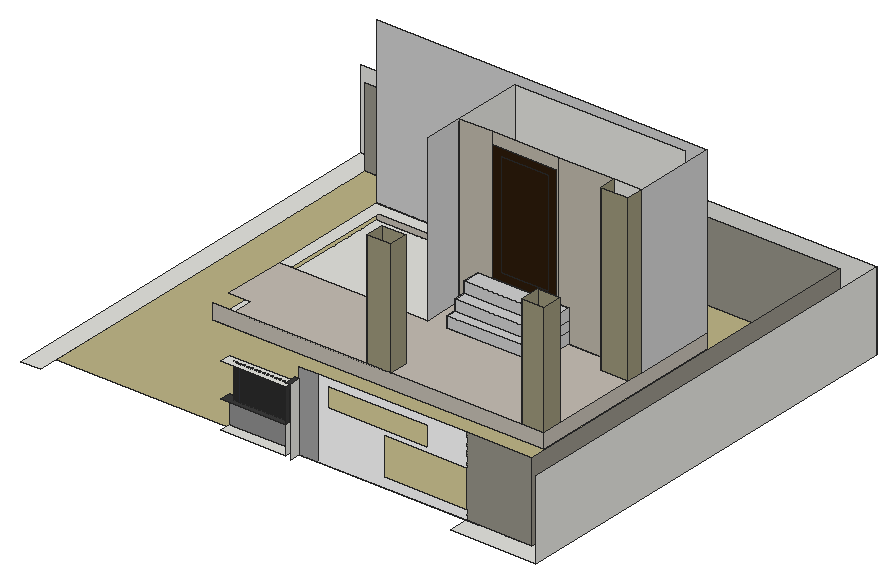
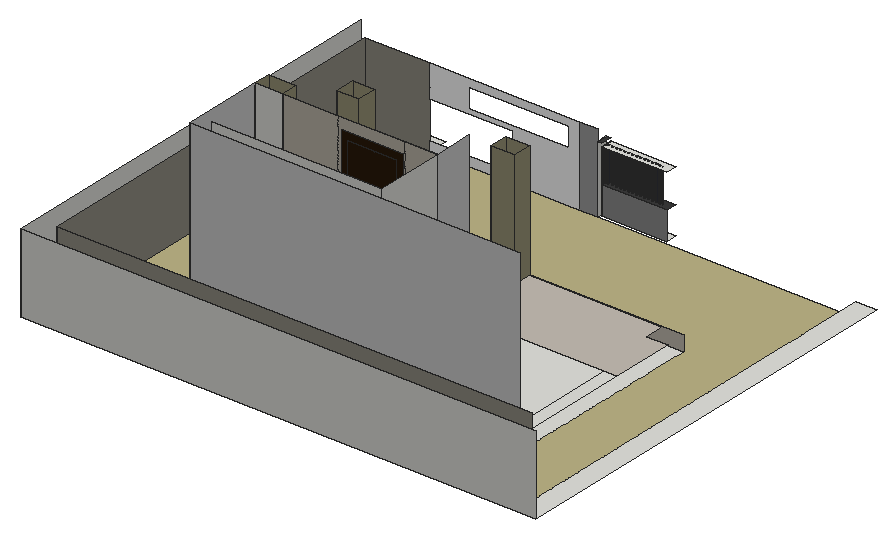
# SketchUp Ruby script. Lengths in inches.
U = 1.inch
M = Sketchup.active_model
def pt(a) = Geom::Point3d.new(a.map { |v| v * U })
def face(e, loops, mat)
  f = e.add_face(loops[0].map { |a| pt(a) })
  loops[1..].each { |l| e.add_face(l.map { |a| pt(a) }).erase! }
  f.material = f.back_material = mat if mat
  f
end
# faces: each face lists its corners as indices into pts; further lists are holes
def faces(e, pts, list, mat = nil) = list.each { |f| face(e, (f[0].is_a?(Array) ? f : [f]).map { |l| l.map { |i| pts[i] } }, mat) }
# xy, xz, yz: faces in a plane at the given z, y or x. An outline is a flat list of corners, or four numbers for a rectangle; further outlines are holes
def ring(l) = l.size == 4 ? [[l[0], l[1]], [l[2], l[1]], [l[2], l[3]], [l[0], l[3]]] : l.each_slice(2).to_a
def flat(e, list, mat, &to3) = list.each { |f| face(e, (f[0].is_a?(Array) ? f : [f]).map { |l| ring(l).map { |u, v| to3.(u, v) } }, mat) }
def xy(e, z, list, mat = nil) = flat(e, list, mat) { |x, y| [x, y, z] }
def xz(e, y, list, mat = nil) = flat(e, list, mat) { |x, z| [x, y, z] }
def yz(e, x, list, mat = nil) = flat(e, list, mat) { |y, z| [x, y, z] }
def lines(e, pts, list) = list.each { |a, b| e.add_line(pt(pts[a]), pt(pts[b])) }
# prism: a flat outline (further loops are holes) pulled along v
def prism(e, loops, v, mat = nil)
  f = face(e, loops, mat); d = Geom::Vector3d.new(v.map { |x| x * U })
  f.pushpull(f.normal.samedirection?(d) ? d.length : -d.length)
end
def box(e, o, s, mat = nil) = prism(e, [[o, [o[0] + s[0], o[1], o[2]], [o[0] + s[0], o[1] + s[1], o[2]], [o[0], o[1] + s[1], o[2]]]], [0, 0, s[2]], mat)
def at(x, y, z, deg = 0) = Geom::Transformation.translation(pt([x, y, z])) * Geom::Transformation.rotation(ORIGIN, Z_AXIS, deg.degrees)
def axes(o, x, y, z) = Geom::Transformation.new([*x, 0, *y, 0, *z, 0, *pt(o).to_a, 1])
def part(name) = M.definitions.add(name)
# library, detail: a bought-in or finely detailed component or shape, given as its bounding box
def library(name, o, s) = part(name).tap { |d| box(d.entities, o, s) }
def detail(e, o, s) = box(e.add_group.entities, o, s)
def put(e, d, t, mat = nil) = e.add_instance(d, t).tap { |i| i.material = mat if mat }
def group(e, t, mat = nil) = e.add_group.tap { |g| g.transformation = t; g.material = mat if mat }.entities
root = M.entities
M.materials.add("[Blinds Vertical Stripe Gray]").color = [160, 160, 160]
M.materials.add("[Blinds Vertical Stripe Gray]1").color = [252, 252, 252]
M.materials.add("[Carrera Marble]").color = [207, 207, 207]
M.materials.add("[Cinder Block]").color = [191, 184, 171]
M.materials.add("[Cladding Siding White]").color = [207, 207, 207]
M.materials.add("[Color M04]").color = [142, 142, 142]
M.materials.add("[Color M07]").color = [58, 58, 58]
M.materials.add("[Field Rectangle Tile]").color = [196, 189, 179]
M.materials.add("[Formica Graystone]").color = [149, 146, 135]
M.materials.add("[Formica Laminate Dark]").color = [50, 53, 60]
M.materials.add("[Stone Coursed Rough]").color = [155, 150, 122]
M.materials.add("[Tile Ceramic Natural]").color = [189, 180, 134]
M.materials.add("[Wood Floor Parquet]").color = [45, 28, 12]
xy(root,0,[[0,96.24,0,408.18,377.8125,408.18,377.8125,96.24,315.3,96.24,315.3,111,363.05,111,363.05,393.42,14.76,393.42,14.76,96.24],[55.77,203.17,297.85,352.92]])
xy(root,0,[[[14.76,111,363.05,393.42],[55.77,203.17,297.85,352.92]]],"[Tile Ceramic Natural]")
xy(root,1.75,[[141.86,102.91,189.5,111]])
xy(root,10.875,[[168.55,203.17,186.24,216.5],[281.86,203.17,297.85,217.98],[55.77,263.99,55.77,352.92,297.85,352.92,297.85,292.92,288.72,292.92,288.72,343.79,64.9,343.79,64.9,263.99],[178.12,264.54,244.68,292.92],[277.86,280.61,288.72,292.92],
  [288.72,280.61,297.85,292.92],[164.37,292.92,288.72,343.79]])
xy(root,10.875,[[71.76,203.17,168.55,203.17,168.55,216.5,186.24,216.5,186.24,203.17,281.86,203.17,281.86,217.98,297.85,217.98,297.85,280.61,277.86,280.61,277.86,292.92,244.68,292.92,244.68,264.54,178.12,264.54,178.12,292.92,164.37,292.92,164.37,263.99,55.77,263.99,55.77,217.98,71.76,217.98]],"[Field Rectangle Tile]")
xy(root,18.65,[[178.12,271.92,244.68,292.92]])
xy(root,18.65,[[178.12,264.54,244.68,271.92]],"[Carrera Marble]")
xy(root,22.1875,[[[141.86,102.91,189.5,111],[144.08,106,143.9,106.02,143.74,106.09,143.6,106.2,143.49,106.34,143.42,106.51,143.4,106.6875,143.42,106.87,143.49,107.03,143.6,107.17,143.74,107.28,143.9,107.35,144.08,107.375,144.26,107.35,144.43,107.28,144.57,107.17,144.68,107.03,144.75,106.87,144.77,106.6875,144.75,106.51,144.68,106.34,144.57,106.2,144.43,106.09,144.26,106.02],[146.96,106,146.78,106.02,146.61,106.09,146.47,106.2,146.36,106.34,146.29,106.51,146.27,106.6875,146.29,106.87,146.36,107.03,146.47,107.17,146.61,107.28,146.78,107.35,146.96,107.375,147.14,107.35,147.3,107.28,147.44,107.17,147.55,107.03,147.62,106.87,147.65,106.6875,147.62,106.51,147.55,106.34,147.44,106.2,147.3,106.09,147.14,106.02],[149.83,106,149.65,106.02,149.49,106.09,149.35,106.2,149.24,106.34,149.17,106.51,149.15,106.6875,149.17,106.87,149.24,107.03,149.35,107.17,149.49,107.28,149.65,107.35,149.83,107.375,150.01,107.35,150.18,107.28,150.32,107.17,150.43,107.03,150.5,106.87,150.52,106.6875,150.5,106.51,150.43,106.34,150.32,106.2,150.18,106.09,150.01,106.02],[152.71,106,152.53,106.02,152.36,106.09,152.22,106.2,152.11,106.34,152.04,106.51,152.02,106.6875,152.04,106.87,152.11,107.03,152.22,107.17,152.36,107.28,152.53,107.35,152.71,107.375,152.89,107.35,153.05,107.28,153.19,107.17,153.3,107.03,153.37,106.87,153.4,106.6875,153.37,106.51,153.3,106.34,153.19,106.2,153.05,106.09,152.89,106.02],[155.58,106,155.4,106.02,155.24,106.09,155.1,106.2,154.99,106.34,154.92,106.51,154.9,106.6875,154.92,106.87,154.99,107.03,155.1,107.17,155.24,107.28,155.4,107.35,155.58,107.375,155.76,107.35,155.93,107.28,156.07,107.17,156.18,107.03,156.25,106.87,156.27,106.6875,156.25,106.51,156.18,106.34,156.07,106.2,155.93,106.09,155.76,106.02],[158.46,106,158.28,106.02,158.11,106.09,157.97,106.2,157.86,106.34,157.79,106.51,157.77,106.6875,157.79,106.87,157.86,107.03,157.97,107.17,158.11,107.28,158.28,107.35,158.46,107.375,158.64,107.35,158.8,107.28,158.94,107.17,159.05,107.03,159.12,106.87,159.15,106.6875,159.12,106.51,159.05,106.34,158.94,106.2,158.8,106.09,158.64,106.02],[161.33,106,161.15,106.02,160.99,106.09,160.85,106.2,160.74,106.34,160.67,106.51,160.65,106.6875,160.67,106.87,160.74,107.03,160.85,107.17,160.99,107.28,161.15,107.35,161.33,107.375,161.51,107.35,161.68,107.28,161.82,107.17,161.93,107.03,162,106.87,162.02,106.6875,162,106.51,161.93,106.34,161.82,106.2,161.68,106.09,161.51,106.02],[164.21,106,164.03,106.02,163.86,106.09,163.72,106.2,163.61,106.34,163.54,106.51,163.52,106.6875,163.54,106.87,163.61,107.03,163.72,107.17,163.86,107.28,164.03,107.35,164.21,107.375,164.39,107.35,164.55,107.28,164.69,107.17,164.8,107.03,164.87,106.87,164.9,106.6875,164.87,106.51,164.8,106.34,164.69,106.2,164.55,106.09,164.39,106.02],[167.08,106,166.9,106.02,166.74,106.09,166.6,106.2,166.49,106.34,166.42,106.51,166.4,106.6875,166.42,106.87,166.49,107.03,166.6,107.17,166.74,107.28,166.9,107.35,167.08,107.375,167.26,107.35,167.43,107.28,167.57,107.17,167.68,107.03,167.75,106.87,167.77,106.6875,167.75,106.51,167.68,106.34,167.57,106.2,167.43,106.09,167.26,106.02],[169.96,106,169.78,106.02,169.61,106.09,169.47,106.2,169.36,106.34,169.29,106.51,169.27,106.6875,169.29,106.87,169.36,107.03,169.47,107.17,169.61,107.28,169.78,107.35,169.96,107.375,170.14,107.35,170.3,107.28,170.44,107.17,170.55,107.03,170.62,106.87,170.65,106.6875,170.62,106.51,170.55,106.34,170.44,106.2,170.3,106.09,170.14,106.02],[172.83,106,172.65,106.02,172.49,106.09,172.35,106.2,172.24,106.34,172.17,106.51,172.15,106.6875,172.17,106.87,172.24,107.03,172.35,107.17,172.49,107.28,172.65,107.35,172.83,107.375,173.01,107.35,173.18,107.28,173.32,107.17,173.43,107.03,173.5,106.87,173.52,106.6875,173.5,106.51,173.43,106.34,173.32,106.2,173.18,106.09,173.01,106.02],[175.71,106,175.53,106.02,175.36,106.09,175.22,106.2,175.11,106.34,175.04,106.51,175.02,106.6875,175.04,106.87,175.11,107.03,175.22,107.17,175.36,107.28,175.53,107.35,175.71,107.375,175.89,107.35,176.05,107.28,176.19,107.17,176.3,107.03,176.37,106.87,176.4,106.6875,176.37,106.51,176.3,106.34,176.19,106.2,176.05,106.09,175.89,106.02],[178.58,106,178.4,106.02,178.24,106.09,178.1,106.2,177.99,106.34,177.92,106.51,177.9,106.6875,177.92,106.87,177.99,107.03,178.1,107.17,178.24,107.28,178.4,107.35,178.58,107.375,178.76,107.35,178.93,107.28,179.07,107.17,179.18,107.03,179.25,106.87,179.27,106.6875,179.25,106.51,179.18,106.34,179.07,106.2,178.93,106.09,178.76,106.02],[181.46,106,181.28,106.02,181.11,106.09,180.97,106.2,180.86,106.34,180.79,106.51,180.77,106.6875,180.79,106.87,180.86,107.03,180.97,107.17,181.11,107.28,181.28,107.35,181.46,107.375,181.64,107.35,181.8,107.28,181.94,107.17,182.05,107.03,182.12,106.87,182.15,106.6875,182.12,106.51,182.05,106.34,181.94,106.2,181.8,106.09,181.64,106.02],[184.52,106,184.34,106.02,184.18,106.09,184.03,106.2,183.92,106.34,183.86,106.51,183.83,106.6875,183.86,106.87,183.92,107.03,184.03,107.17,184.18,107.28,184.34,107.35,184.52,107.375,184.7,107.35,184.86,107.28,185.01,107.17,185.12,107.03,185.18,106.87,185.21,106.6875,185.18,106.51,185.12,106.34,185.01,106.2,184.86,106.09,184.7,106.02],[187.96,106,187.78,106.02,187.61,106.09,187.47,106.2,187.36,106.34,187.29,106.51,187.27,106.6875,187.29,106.87,187.36,107.03,187.47,107.17,187.61,107.28,187.78,107.35,187.96,107.375,188.14,107.35,188.3,107.28,188.44,107.17,188.55,107.03,188.62,106.87,188.65,106.6875,188.62,106.51,188.55,106.34,188.44,106.2,188.3,106.09,188.14,106.02]]],"[Color M07]")
xy(root,26.42,[[178.12,280.29,244.68,292.92]])
xy(root,26.42,[[178.12,271.92,244.68,280.29]],"[Carrera Marble]")
xy(root,34.61,[[178.12,280.29,244.68,292.92]],"[Carrera Marble]")
xy(root,47.21,[[[141.86,102.91,189.5,111],[144.08,106,144.26,106.02,144.43,106.09,144.57,106.2,144.68,106.34,144.75,106.51,144.77,106.6875,144.75,106.87,144.68,107.03,144.57,107.17,144.43,107.28,144.26,107.35,144.08,107.375,143.9,107.35,143.74,107.28,143.6,107.17,143.49,107.03,143.42,106.87,143.4,106.6875,143.42,106.51,143.49,106.34,143.6,106.2,143.74,106.09,143.9,106.02],[146.96,106,147.14,106.02,147.3,106.09,147.44,106.2,147.55,106.34,147.62,106.51,147.65,106.6875,147.62,106.87,147.55,107.03,147.44,107.17,147.3,107.28,147.14,107.35,146.96,107.375,146.78,107.35,146.61,107.28,146.47,107.17,146.36,107.03,146.29,106.87,146.27,106.6875,146.29,106.51,146.36,106.34,146.47,106.2,146.61,106.09,146.78,106.02],[149.83,106,150.01,106.02,150.18,106.09,150.32,106.2,150.43,106.34,150.5,106.51,150.52,106.6875,150.5,106.87,150.43,107.03,150.32,107.17,150.18,107.28,150.01,107.35,149.83,107.375,149.65,107.35,149.49,107.28,149.35,107.17,149.24,107.03,149.17,106.87,149.15,106.6875,149.17,106.51,149.24,106.34,149.35,106.2,149.49,106.09,149.65,106.02],[152.71,106,152.89,106.02,153.05,106.09,153.19,106.2,153.3,106.34,153.37,106.51,153.4,106.6875,153.37,106.87,153.3,107.03,153.19,107.17,153.05,107.28,152.89,107.35,152.71,107.375,152.53,107.35,152.36,107.28,152.22,107.17,152.11,107.03,152.04,106.87,152.02,106.6875,152.04,106.51,152.11,106.34,152.22,106.2,152.36,106.09,152.53,106.02],[187.96,106,188.14,106.02,188.3,106.09,188.44,106.2,188.55,106.34,188.62,106.51,188.65,106.6875,188.62,106.87,188.55,107.03,188.44,107.17,188.3,107.28,188.14,107.35,187.96,107.375,187.78,107.35,187.61,107.28,187.47,107.17,187.36,107.03,187.29,106.87,187.27,106.6875,187.29,106.51,187.36,106.34,187.47,106.2,187.61,106.09,187.78,106.02],[184.52,106,184.7,106.02,184.86,106.09,185.01,106.2,185.12,106.34,185.18,106.51,185.21,106.6875,185.18,106.87,185.12,107.03,185.01,107.17,184.86,107.28,184.7,107.35,184.52,107.375,184.34,107.35,184.18,107.28,184.03,107.17,183.92,107.03,183.86,106.87,183.83,106.6875,183.86,106.51,183.92,106.34,184.03,106.2,184.18,106.09,184.34,106.02],[181.46,106,181.64,106.02,181.8,106.09,181.94,106.2,182.05,106.34,182.12,106.51,182.15,106.6875,182.12,106.87,182.05,107.03,181.94,107.17,181.8,107.28,181.64,107.35,181.46,107.375,181.28,107.35,181.11,107.28,180.97,107.17,180.86,107.03,180.79,106.87,180.77,106.6875,180.79,106.51,180.86,106.34,180.97,106.2,181.11,106.09,181.28,106.02],[178.58,106,178.76,106.02,178.93,106.09,179.07,106.2,179.18,106.34,179.25,106.51,179.27,106.6875,179.25,106.87,179.18,107.03,179.07,107.17,178.93,107.28,178.76,107.35,178.58,107.375,178.4,107.35,178.24,107.28,178.1,107.17,177.99,107.03,177.92,106.87,177.9,106.6875,177.92,106.51,177.99,106.34,178.1,106.2,178.24,106.09,178.4,106.02],[175.71,106,175.89,106.02,176.05,106.09,176.19,106.2,176.3,106.34,176.37,106.51,176.4,106.6875,176.37,106.87,176.3,107.03,176.19,107.17,176.05,107.28,175.89,107.35,175.71,107.375,175.53,107.35,175.36,107.28,175.22,107.17,175.11,107.03,175.04,106.87,175.02,106.6875,175.04,106.51,175.11,106.34,175.22,106.2,175.36,106.09,175.53,106.02],[172.83,106,173.01,106.02,173.18,106.09,173.32,106.2,173.43,106.34,173.5,106.51,173.52,106.6875,173.5,106.87,173.43,107.03,173.32,107.17,173.18,107.28,173.01,107.35,172.83,107.375,172.65,107.35,172.49,107.28,172.35,107.17,172.24,107.03,172.17,106.87,172.15,106.6875,172.17,106.51,172.24,106.34,172.35,106.2,172.49,106.09,172.65,106.02],[169.96,106,170.14,106.02,170.3,106.09,170.44,106.2,170.55,106.34,170.62,106.51,170.65,106.6875,170.62,106.87,170.55,107.03,170.44,107.17,170.3,107.28,170.14,107.35,169.96,107.375,169.78,107.35,169.61,107.28,169.47,107.17,169.36,107.03,169.29,106.87,169.27,106.6875,169.29,106.51,169.36,106.34,169.47,106.2,169.61,106.09,169.78,106.02],[167.08,106,167.26,106.02,167.43,106.09,167.57,106.2,167.68,106.34,167.75,106.51,167.77,106.6875,167.75,106.87,167.68,107.03,167.57,107.17,167.43,107.28,167.26,107.35,167.08,107.375,166.9,107.35,166.74,107.28,166.6,107.17,166.49,107.03,166.42,106.87,166.4,106.6875,166.42,106.51,166.49,106.34,166.6,106.2,166.74,106.09,166.9,106.02],[164.21,106,164.39,106.02,164.55,106.09,164.69,106.2,164.8,106.34,164.87,106.51,164.9,106.6875,164.87,106.87,164.8,107.03,164.69,107.17,164.55,107.28,164.39,107.35,164.21,107.375,164.03,107.35,163.86,107.28,163.72,107.17,163.61,107.03,163.54,106.87,163.52,106.6875,163.54,106.51,163.61,106.34,163.72,106.2,163.86,106.09,164.03,106.02],[161.33,106,161.51,106.02,161.68,106.09,161.82,106.2,161.93,106.34,162,106.51,162.02,106.6875,162,106.87,161.93,107.03,161.82,107.17,161.68,107.28,161.51,107.35,161.33,107.375,161.15,107.35,160.99,107.28,160.85,107.17,160.74,107.03,160.67,106.87,160.65,106.6875,160.67,106.51,160.74,106.34,160.85,106.2,160.99,106.09,161.15,106.02],[158.46,106,158.64,106.02,158.8,106.09,158.94,106.2,159.05,106.34,159.12,106.51,159.15,106.6875,159.12,106.87,159.05,107.03,158.94,107.17,158.8,107.28,158.64,107.35,158.46,107.375,158.28,107.35,158.11,107.28,157.97,107.17,157.86,107.03,157.79,106.87,157.77,106.6875,157.79,106.51,157.86,106.34,157.97,106.2,158.11,106.09,158.28,106.02],[155.58,106,155.76,106.02,155.93,106.09,156.07,106.2,156.18,106.34,156.25,106.51,156.27,106.6875,156.25,106.87,156.18,107.03,156.07,107.17,155.93,107.28,155.76,107.35,155.58,107.375,155.4,107.35,155.24,107.28,155.1,107.17,154.99,107.03,154.92,106.87,154.9,106.6875,154.92,106.51,154.99,106.34,155.1,106.2,155.24,106.09,155.4,106.02]]])
xy(root,49.625,[[189.5,102.91,192.64,111]],"[Color M07]")
xz(root,111,[[192.64,0,206.19,57.8125]],"[Blinds Vertical Stripe Gray]")
xz(root,111,[[[206.19,0,206.19,57.8125,315.3,57.8125,315.3,34.41,254.71,34.41,254.71,7.1,315.3,7.1,315.3,0],[213.78,37.78,286.85,52.34]]],"[Blinds Vertical Stripe Gray]1")
xz(root,111,[[141.86,1.75,189.5,22.1875]],"[Color M04]")
xz(root,111,[[315.3,0,363.05,57.8125]],"[Formica Graystone]")
xz(root,203.17,[[55.77,0,297.85,10.875]],"[Field Rectangle Tile]")
xz(root,203.17,[[168.55,10.875,186.24,95.36],[281.86,10.875,297.85,92.87]],"[Stone Coursed Rough]")
xz(root,216.5,[[168.55,10.875,186.24,95.36]],"[Stone Coursed Rough]")
xz(root,217.98,[[281.86,10.875,297.85,92.87]],"[Stone Coursed Rough]")
xz(root,264.54,[[178.12,10.875,244.68,18.65]],"[Carrera Marble]")
xz(root,271.92,[[178.12,18.65,244.68,26.42]],"[Carrera Marble]")
xz(root,280.29,[[178.12,26.42,244.68,34.61]],"[Carrera Marble]")
xz(root,280.61,[[277.86,10.875,297.85,130.875]],"[Stone Coursed Rough]")
xz(root,292.92,[[178.12,10.875,244.68,18.65],[277.86,10.875,297.85,130.875],[178.12,18.65,244.68,26.42],[178.12,26.42,244.68,34.61]])
xz(root,292.92,[[164.37,10.875,178.12,10.875,178.12,34.61,188.27,34.61,188.27,130.875,164.37,130.875],[244.68,10.875,277.86,10.875,277.86,130.875,237.125,130.875,237.125,34.61,244.68,34.61],[188.27,34.61,189.12,34.61,189.12,122.36,235.43,122.36,235.43,34.61,237.125,34.61,237.125,130.875,188.27,130.875]],"[Cinder Block]")
xz(root,292.92,[[[189.12,34.61,235.43,122.36],[194.54,40.04,230,116.94]],[194.54,40.04,230,116.94]],"[Wood Floor Parquet]")
xz(root,343.79,[[164.37,10.875,288.72,130.875]])
xz(root,352.92,[[55.77,10.875,297.85,130.875]],"[Cladding Siding White]")
xz(root,352.92,[[55.77,0,297.85,10.875]],"[Field Rectangle Tile]")
xz(root,393.42,[[14.76,0,363.05,57.8125]],"[Formica Graystone]")
xz(root,408.18,[[0,0,377.8125,57.8125]])
yz(root,164.37,[[292.92,10.875,343.79,130.875]])
yz(root,164.37,[[263.99,10.875,292.92,130.875]],"[Cladding Siding White]")
yz(root,168.55,[[203.17,10.875,216.5,95.36]],"[Stone Coursed Rough]")
yz(root,178.12,[[264.54,10.875,292.92,18.65],[271.92,18.65,292.92,26.42],[280.29,26.42,292.92,34.61]],"[Carrera Marble]")
yz(root,186.24,[[203.17,10.875,216.5,95.36]],"[Stone Coursed Rough]")
yz(root,189.5,[[102.91,1.75,111,22.1875]])
yz(root,189.5,[[102.91,22.1875,111,47.21]],"[Color M07]")
yz(root,192.64,[[102.91,0,111,49.625]])
yz(root,244.68,[[264.54,10.875,292.92,18.65],[271.92,18.65,292.92,26.42],[280.29,26.42,292.92,34.61]],"[Carrera Marble]")
yz(root,277.86,[[280.61,10.875,292.92,130.875]],"[Stone Coursed Rough]")
yz(root,281.86,[[203.17,10.875,217.98,92.87]],"[Stone Coursed Rough]")
yz(root,297.85,[[292.92,10.875,352.92,130.875]],"[Cladding Siding White]")
yz(root,297.85,[[203.17,0,352.92,10.875]],"[Field Rectangle Tile]")
yz(root,297.85,[[203.17,10.875,217.98,92.87],[280.61,10.875,292.92,130.875]],"[Stone Coursed Rough]")
yz(root,363.05,[[111,0,393.42,57.8125]],"[Formica Graystone]")
yz(root,377.8125,[[96.24,0,408.18,57.8125]])
p = [[150.52,106.6875,22.1875],[150.5,106.87,22.1875],[150.5,106.87,47.21],[150.52,106.6875,47.21],[152.04,106.87,22.1875],[152.02,106.6875,22.1875],
  [152.02,106.6875,47.21],[152.04,106.87,47.21],[153.4,106.6875,22.1875],[153.37,106.87,22.1875],[153.37,106.87,47.21],[153.4,106.6875,47.21],
  [154.92,106.87,22.1875],[154.9,106.6875,22.1875],[154.9,106.6875,47.21],[154.92,106.87,47.21],[156.27,106.6875,22.1875],[156.25,106.87,22.1875],
  [156.25,106.87,47.21],[156.27,106.6875,47.21],[157.79,106.87,22.1875],[157.77,106.6875,22.1875],[157.77,106.6875,47.21],[157.79,106.87,47.21],
  [159.15,106.6875,22.1875],[159.12,106.87,22.1875],[159.12,106.87,47.21],[159.15,106.6875,47.21],[160.67,106.87,22.1875],[160.65,106.6875,22.1875],
  [160.65,106.6875,47.21],[160.67,106.87,47.21],[162.02,106.6875,22.1875],[162,106.87,22.1875],[162,106.87,47.21],[162.02,106.6875,47.21],
  [163.54,106.87,22.1875],[163.52,106.6875,22.1875],[163.52,106.6875,47.21],[163.54,106.87,47.21],[164.9,106.6875,22.1875],[164.87,106.87,22.1875],
  [164.87,106.87,47.21],[164.9,106.6875,47.21],[166.42,106.87,22.1875],[166.4,106.6875,22.1875],[166.4,106.6875,47.21],[166.42,106.87,47.21],
  [167.77,106.6875,22.1875],[167.75,106.87,22.1875],[167.75,106.87,47.21],[167.77,106.6875,47.21],[169.29,106.87,22.1875],[169.27,106.6875,22.1875],
  [169.27,106.6875,47.21],[169.29,106.87,47.21],[170.65,106.6875,22.1875],[170.62,106.87,22.1875],[170.62,106.87,47.21],[170.65,106.6875,47.21],
  [172.17,106.87,22.1875],[172.15,106.6875,22.1875],[172.15,106.6875,47.21],[172.17,106.87,47.21],[173.52,106.6875,22.1875],[173.5,106.87,22.1875],
  [173.5,106.87,47.21],[173.52,106.6875,47.21],[175.04,106.87,22.1875],[175.02,106.6875,22.1875],[175.02,106.6875,47.21],[175.04,106.87,47.21],
  [176.4,106.6875,22.1875],[176.37,106.87,22.1875],[176.37,106.87,47.21],[176.4,106.6875,47.21],[177.92,106.87,22.1875],[177.9,106.6875,22.1875],
  [177.9,106.6875,47.21],[177.92,106.87,47.21],[179.27,106.6875,22.1875],[179.25,106.87,22.1875],[179.25,106.87,47.21],[179.27,106.6875,47.21],
  [180.79,106.87,22.1875],[180.77,106.6875,22.1875],[180.77,106.6875,47.21],[180.79,106.87,47.21],[182.15,106.6875,22.1875],[182.12,106.87,22.1875],
  [182.12,106.87,47.21],[182.15,106.6875,47.21],[183.86,106.87,22.1875],[183.83,106.6875,22.1875],[183.83,106.6875,47.21],[183.86,106.87,47.21],
  [185.21,106.6875,22.1875],[185.18,106.87,22.1875],[185.18,106.87,47.21],[185.21,106.6875,47.21],[187.29,106.87,22.1875],[187.27,106.6875,22.1875],
  [187.27,106.6875,47.21],[187.29,106.87,47.21],[188.65,106.6875,22.1875],[188.62,106.87,22.1875],[188.62,106.87,47.21],[188.65,106.6875,47.21],
  [147.62,106.87,22.1875],[147.55,107.03,22.1875],[147.55,107.03,47.21],[147.62,106.87,47.21],[149.24,107.03,22.1875],[149.17,106.87,22.1875],
  [149.17,106.87,47.21],[149.24,107.03,47.21],[150.43,107.03,22.1875],[150.43,107.03,47.21],[152.11,107.03,22.1875],[152.11,107.03,47.21],
  [153.3,107.03,22.1875],[153.3,107.03,47.21],[154.99,107.03,22.1875],[154.99,107.03,47.21],[156.18,107.03,22.1875],[156.18,107.03,47.21],
  [157.86,107.03,22.1875],[157.86,107.03,47.21],[159.05,107.03,22.1875],[159.05,107.03,47.21],[160.74,107.03,22.1875],[160.74,107.03,47.21],
  [161.93,107.03,22.1875],[161.93,107.03,47.21],[163.61,107.03,22.1875],[163.61,107.03,47.21],[164.8,107.03,22.1875],[164.8,107.03,47.21],
  [166.49,107.03,22.1875],[166.49,107.03,47.21],[167.68,107.03,22.1875],[167.68,107.03,47.21],[169.36,107.03,22.1875],[169.36,107.03,47.21],
  [170.55,107.03,22.1875],[170.55,107.03,47.21],[172.24,107.03,22.1875],[172.24,107.03,47.21],[173.43,107.03,22.1875],[173.43,107.03,47.21],
  [175.11,107.03,22.1875],[175.11,107.03,47.21],[176.3,107.03,22.1875],[176.3,107.03,47.21],[177.99,107.03,22.1875],[177.99,107.03,47.21],
  [179.18,107.03,22.1875],[179.18,107.03,47.21],[180.86,107.03,22.1875],[180.86,107.03,47.21],[182.05,107.03,22.1875],[182.05,107.03,47.21],
  [183.92,107.03,22.1875],[183.92,107.03,47.21],[185.12,107.03,22.1875],[185.12,107.03,47.21],[187.36,107.03,22.1875],[187.36,107.03,47.21],
  [188.55,107.03,22.1875],[188.55,107.03,47.21],[147.44,107.17,22.1875],[147.44,107.17,47.21],[149.35,107.17,22.1875],[149.35,107.17,47.21],
  [150.32,107.17,22.1875],[150.32,107.17,47.21],[152.22,107.17,22.1875],[152.22,107.17,47.21],[153.19,107.17,22.1875],[153.19,107.17,47.21],
  [155.1,107.17,22.1875],[155.1,107.17,47.21],[156.07,107.17,22.1875],[156.07,107.17,47.21],[157.97,107.17,22.1875],[157.97,107.17,47.21],
  [158.94,107.17,22.1875],[158.94,107.17,47.21],[160.85,107.17,22.1875],[160.85,107.17,47.21],[161.82,107.17,22.1875],[161.82,107.17,47.21],
  [163.72,107.17,22.1875],[163.72,107.17,47.21],[164.69,107.17,22.1875],[164.69,107.17,47.21],[166.6,107.17,22.1875],[166.6,107.17,47.21],
  [167.57,107.17,22.1875],[167.57,107.17,47.21],[169.47,107.17,22.1875],[169.47,107.17,47.21],[170.44,107.17,22.1875],[170.44,107.17,47.21],
  [172.35,107.17,22.1875],[172.35,107.17,47.21],[173.32,107.17,22.1875],[173.32,107.17,47.21],[175.22,107.17,22.1875],[175.22,107.17,47.21],
  [176.19,107.17,22.1875],[176.19,107.17,47.21],[178.1,107.17,22.1875],[178.1,107.17,47.21],[179.07,107.17,22.1875],[179.07,107.17,47.21],
  [180.97,107.17,22.1875],[180.97,107.17,47.21],[181.94,107.17,22.1875],[181.94,107.17,47.21],[184.03,107.17,22.1875],[184.03,107.17,47.21],
  [185.01,107.17,22.1875],[185.01,107.17,47.21],[187.47,107.17,22.1875],[187.47,107.17,47.21],[188.44,107.17,22.1875],[188.44,107.17,47.21],
  [147.3,107.28,22.1875],[147.3,107.28,47.21],[149.49,107.28,22.1875],[149.49,107.28,47.21],[150.18,107.28,22.1875],[150.18,107.28,47.21],
  [152.36,107.28,22.1875],[152.36,107.28,47.21],[153.05,107.28,22.1875],[153.05,107.28,47.21],[155.24,107.28,22.1875],[155.24,107.28,47.21],
  [155.93,107.28,22.1875],[155.93,107.28,47.21],[158.11,107.28,22.1875],[158.11,107.28,47.21],[158.8,107.28,22.1875],[158.8,107.28,47.21],
  [160.99,107.28,22.1875],[160.99,107.28,47.21],[161.68,107.28,22.1875],[161.68,107.28,47.21],[163.86,107.28,22.1875],[163.86,107.28,47.21],
  [164.55,107.28,22.1875],[164.55,107.28,47.21],[166.74,107.28,22.1875],[166.74,107.28,47.21],[167.43,107.28,22.1875],[167.43,107.28,47.21],
  [169.61,107.28,22.1875],[169.61,107.28,47.21],[170.3,107.28,22.1875],[170.3,107.28,47.21],[172.49,107.28,22.1875],[172.49,107.28,47.21],
  [173.18,107.28,22.1875],[173.18,107.28,47.21],[175.36,107.28,22.1875],[175.36,107.28,47.21],[176.05,107.28,22.1875],[176.05,107.28,47.21],
  [178.24,107.28,22.1875],[178.24,107.28,47.21],[178.93,107.28,22.1875],[178.93,107.28,47.21],[181.11,107.28,22.1875],[181.11,107.28,47.21],
  [181.8,107.28,22.1875],[181.8,107.28,47.21],[184.18,107.28,22.1875],[184.18,107.28,47.21],[184.86,107.28,22.1875],[184.86,107.28,47.21],
  [187.61,107.28,22.1875],[187.61,107.28,47.21],[188.3,107.28,22.1875],[188.3,107.28,47.21],[149.65,107.35,22.1875],[149.65,107.35,47.21],
  [150.01,107.35,22.1875],[150.01,107.35,47.21],[152.53,107.35,22.1875],[152.53,107.35,47.21],[152.89,107.35,22.1875],[152.89,107.35,47.21],
  [155.4,107.35,22.1875],[155.4,107.35,47.21],[155.76,107.35,22.1875],[155.76,107.35,47.21],[158.28,107.35,22.1875],[158.28,107.35,47.21],
  [158.64,107.35,22.1875],[158.64,107.35,47.21],[161.15,107.35,22.1875],[161.15,107.35,47.21],[161.51,107.35,22.1875],[161.51,107.35,47.21],
  [164.03,107.35,22.1875],[164.03,107.35,47.21],[164.39,107.35,22.1875],[164.39,107.35,47.21],[166.9,107.35,22.1875],[166.9,107.35,47.21],
  [167.26,107.35,22.1875],[167.26,107.35,47.21],[169.78,107.35,22.1875],[169.78,107.35,47.21],[170.14,107.35,22.1875],[170.14,107.35,47.21],
  [172.65,107.35,22.1875],[172.65,107.35,47.21],[173.01,107.35,22.1875],[173.01,107.35,47.21],[175.53,107.35,22.1875],[175.53,107.35,47.21],
  [175.89,107.35,22.1875],[175.89,107.35,47.21],[178.4,107.35,22.1875],[178.4,107.35,47.21],[178.76,107.35,22.1875],[178.76,107.35,47.21],
  [181.28,107.35,22.1875],[181.28,107.35,47.21],[181.64,107.35,22.1875],[181.64,107.35,47.21],[184.34,107.35,22.1875],[184.34,107.35,47.21],
  [184.7,107.35,22.1875],[184.7,107.35,47.21],[187.78,107.35,22.1875],[187.78,107.35,47.21],[188.14,107.35,22.1875],[188.14,107.35,47.21],
  [149.83,107.375,22.1875],[149.83,107.375,47.21],[152.71,107.375,22.1875],[152.71,107.375,47.21],[155.58,107.375,22.1875],[155.58,107.375,47.21],
  [158.46,107.375,22.1875],[158.46,107.375,47.21],[161.33,107.375,22.1875],[161.33,107.375,47.21],[164.21,107.375,22.1875],[164.21,107.375,47.21],
  [167.08,107.375,22.1875],[167.08,107.375,47.21],[169.96,107.375,22.1875],[169.96,107.375,47.21],[172.83,107.375,22.1875],[172.83,107.375,47.21],
  [175.71,107.375,22.1875],[175.71,107.375,47.21],[178.58,107.375,22.1875],[178.58,107.375,47.21],[181.46,107.375,22.1875],[181.46,107.375,47.21],
  [184.52,107.375,22.1875],[184.52,107.375,47.21],[187.96,107.375,22.1875],[187.96,107.375,47.21]]
faces(root,p,[[0,1,2,3],[4,5,6,7],[8,9,10,11],[12,13,14,15],[16,17,18,19],[20,21,22,23],[24,25,26,27],[28,29,30,31],
  [32,33,34,35],[36,37,38,39],[40,41,42,43],[44,45,46,47],[48,49,50,51],[52,53,54,55],[56,57,58,59],[60,61,62,63],
  [64,65,66,67],[68,69,70,71],[72,73,74,75],[76,77,78,79],[80,81,82,83],[84,85,86,87],[88,89,90,91],[92,93,94,95],
  [96,97,98,99],[100,101,102,103],[104,105,106,107],[108,109,110,111],[112,113,114,115],[1,116,117,2],[118,4,7,119],[9,120,121,10],
  [122,12,15,123],[17,124,125,18],[126,20,23,127],[25,128,129,26],[130,28,31,131],[33,132,133,34],[134,36,39,135],[41,136,137,42],
  [138,44,47,139],[49,140,141,50],[142,52,55,143],[57,144,145,58],[146,60,63,147],[65,148,149,66],[150,68,71,151],[73,152,153,74],
  [154,76,79,155],[81,156,157,82],[158,84,87,159],[89,160,161,90],[162,92,95,163],[97,164,165,98],[166,100,103,167],[105,168,169,106],
  [109,170,171,110],[172,112,115,173],[116,174,175,117],[176,118,119,177],[120,178,179,121],[180,122,123,181],[124,182,183,125],[184,126,127,185],
  [128,186,187,129],[188,130,131,189],[132,190,191,133],[192,134,135,193],[136,194,195,137],[196,138,139,197],[140,198,199,141],[200,142,143,201],
  [144,202,203,145],[204,146,147,205],[148,206,207,149],[208,150,151,209],[152,210,211,153],[212,154,155,213],[156,214,215,157],[216,158,159,217],
  [160,218,219,161],[220,162,163,221],[164,222,223,165],[224,166,167,225],[168,226,227,169],[170,228,229,171],[230,172,173,231],[174,232,233,175],
  [234,176,177,235],[178,236,237,179],[238,180,181,239],[182,240,241,183],[242,184,185,243],[186,244,245,187],[246,188,189,247],[190,248,249,191],
  [250,192,193,251],[194,252,253,195],[254,196,197,255],[198,256,257,199],[258,200,201,259],[202,260,261,203],[262,204,205,263],[206,264,265,207],
  [266,208,209,267],[210,268,269,211],[270,212,213,271],[214,272,273,215],[274,216,217,275],[218,276,277,219],[278,220,221,279],[222,280,281,223],
  [282,224,225,283],[226,284,285,227],[286,230,231,287],[232,288,289,233],[290,234,235,291],[236,292,293,237],[294,238,239,295],[240,296,297,241],
  [298,242,243,299],[244,300,301,245],[302,246,247,303],[248,304,305,249],[306,250,251,307],[252,308,309,253],[310,254,255,311],[256,312,313,257],
  [314,258,259,315],[260,316,317,261],[318,262,263,319],[264,320,321,265],[322,266,267,323],[268,324,325,269],[326,270,271,327],[272,328,329,273],
  [330,274,275,331],[276,332,333,277],[334,278,279,335],[280,336,337,281],[338,282,283,339],[284,340,341,285],[342,286,287,343],[288,342,343,289],
  [344,290,291,345],[292,344,345,293],[346,294,295,347],[296,346,347,297],[348,298,299,349],[300,348,349,301],[350,302,303,351],[304,350,351,305],
  [352,306,307,353],[308,352,353,309],[354,310,311,355],[312,354,355,313],[356,314,315,357],[316,356,357,317],[358,318,319,359],[320,358,359,321],
  [360,322,323,361],[324,360,361,325],[362,326,327,363],[328,362,363,329],[364,330,331,365],[332,364,365,333],[366,334,335,367],[336,366,367,337],
  [368,338,339,369],[340,368,369,341]],"[Formica Laminate Dark]")
